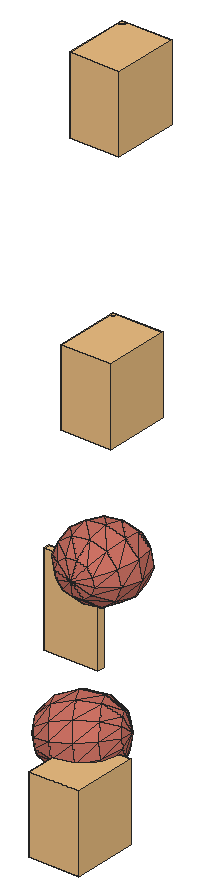
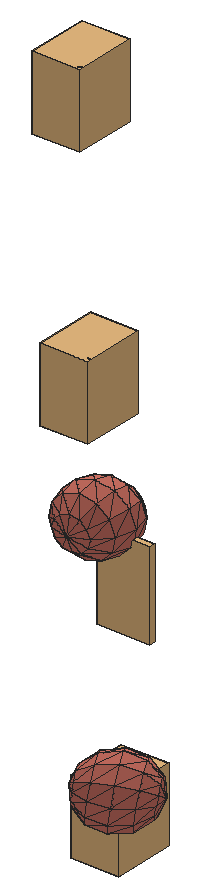
# SketchUp Ruby script. Lengths in inches.
U = 1.inch
M = Sketchup.active_model
def pt(a) = Geom::Point3d.new(a.map { |v| v * U })
def face(e, loops, mat)
  f = e.add_face(loops[0].map { |a| pt(a) })
  loops[1..].each { |l| e.add_face(l.map { |a| pt(a) }).erase! }
  f.material = f.back_material = mat if mat
  f
end
# faces: each face lists its corners as indices into pts; further lists are holes
def faces(e, pts, list, mat = nil) = list.each { |f| face(e, (f[0].is_a?(Array) ? f : [f]).map { |l| l.map { |i| pts[i] } }, mat) }
# xy, xz, yz: faces in a plane at the given z, y or x. An outline is a flat list of corners, or four numbers for a rectangle; further outlines are holes
def ring(l) = l.size == 4 ? [[l[0], l[1]], [l[2], l[1]], [l[2], l[3]], [l[0], l[3]]] : l.each_slice(2).to_a
def flat(e, list, mat, &to3) = list.each { |f| face(e, (f[0].is_a?(Array) ? f : [f]).map { |l| ring(l).map { |u, v| to3.(u, v) } }, mat) }
def xy(e, z, list, mat = nil) = flat(e, list, mat) { |x, y| [x, y, z] }
def xz(e, y, list, mat = nil) = flat(e, list, mat) { |x, z| [x, y, z] }
def yz(e, x, list, mat = nil) = flat(e, list, mat) { |y, z| [x, y, z] }
def lines(e, pts, list) = list.each { |a, b| e.add_line(pt(pts[a]), pt(pts[b])) }
# prism: a flat outline (further loops are holes) pulled along v
def prism(e, loops, v, mat = nil)
  f = face(e, loops, mat); d = Geom::Vector3d.new(v.map { |x| x * U })
  f.pushpull(f.normal.samedirection?(d) ? d.length : -d.length)
end
def box(e, o, s, mat = nil) = prism(e, [[o, [o[0] + s[0], o[1], o[2]], [o[0] + s[0], o[1] + s[1], o[2]], [o[0], o[1] + s[1], o[2]]]], [0, 0, s[2]], mat)
def at(x, y, z, deg = 0) = Geom::Transformation.translation(pt([x, y, z])) * Geom::Transformation.rotation(ORIGIN, Z_AXIS, deg.degrees)
def axes(o, x, y, z) = Geom::Transformation.new([*x, 0, *y, 0, *z, 0, *pt(o).to_a, 1])
def part(name) = M.definitions.add(name)
# library, detail: a bought-in or finely detailed component or shape, given as its bounding box
def library(name, o, s) = part(name).tap { |d| box(d.entities, o, s) }
def detail(e, o, s) = box(e.add_group.entities, o, s)
def put(e, d, t, mat = nil) = e.add_instance(d, t).tap { |i| i.material = mat if mat }
def group(e, t, mat = nil) = e.add_group.tap { |g| g.transformation = t; g.material = mat if mat }.entities
root = M.entities
M.materials.add("green").color = [174, 139, 102]
M.materials.add("vio").color = [206, 114, 100]
c1 = library("3DGeom~127_Defintion",[-35.65,-500,-298.26],[71.3,1000,596.52])
c2 = part("3DGeom~128_Defintion")
p = [[1.79,-469.7,-298.26],[1.7,-500,-240.6],[-27.6,-477.32,-283.92],[31.13,-477.23,-283.76],[1.7,-500,-240.6],[1.79,-469.7,-298.26],
  [1.79,-469.7,-298.26],[-27.6,-477.32,-283.92],[-15.17,-471.75,-294.44],[31.13,-477.23,-283.76],[1.79,-469.7,-298.26],[18.74,-471.7,-294.35],
  [-27.6,-477.32,-283.92],[1.7,-500,-240.6],[-27.65,-492.47,-255.09],[-27.6,-477.32,-283.92],[-27.65,-492.47,-255.09],[-32.17,-484.9,-269.52],
  [31.09,-492.38,-254.93],[1.7,-500,-240.6],[31.13,-477.23,-283.76],[31.09,-492.38,-254.93],[31.13,-477.23,-283.76],[35.65,-484.8,-269.34],
  [1.7,-500,-240.6],[-15.25,-498,-244.5],[-27.65,-492.47,-255.09],[1.7,-500,-240.6],[31.09,-492.38,-254.93],[18.66,-497.94,-244.41],
  [-1.83,497.78,298.26],[-1.65,500,230.49],[-18.62,499.82,234.98],[-1.83,497.78,298.26],[15.29,499.875,235.07],[-1.65,500,230.49],
  [-1.83,497.78,298.26],[-18.62,499.82,234.98],[-31.0625,499.4,247.35],[-1.83,497.78,298.26],[27.67,499.49,247.51],[15.29,499.875,235.07],
  [-1.83,497.78,298.26],[-31.0625,499.4,247.35],[-35.65,498.84,264.28],[-1.83,497.78,298.26],[32.17,498.94,264.47],[27.67,499.49,247.51],
  [-1.83,497.78,298.26],[-35.65,498.84,264.28],[-31.15,498.29,281.24],[-1.83,497.78,298.26],[27.58,498.375,281.4],[32.17,498.94,264.47],
  [-1.83,497.78,298.26],[-31.15,498.29,281.24],[-18.77,497.9,293.67],[-1.83,497.78,298.26],[15.14,497.95,293.77],[27.58,498.375,281.4]]
faces(c2.entities,p,[[0,1,2],[3,4,5],[6,7,8],[9,10,11],[12,13,14],[15,16,17],[18,19,20],[21,22,23],
  [24,25,26],[27,28,29],[30,31,32],[33,34,35],[36,37,38],[39,40,41],[42,43,44],[45,46,47],
  [48,49,50],[51,52,53],[54,55,56],[57,58,59]],"green")
c3 = part("3DGeom~230_Defintion")
p = [[-248.9,29.76,-432.23],[1.27,34.79,-498.32],[1.59,-181.375,-452.05],[251.38,-156.7,-390.8125],[251.1,30.51,-430.88],[-249.48,208.89,-356.66],
  [0.6,241.64,-411.0625],[-249.48,208.89,-356.66],[-248.62,-157.45,-392.16],[1.49,-348.94,-284.65],[251.29,-301.82,-245.84],[-248.62,-157.45,-392.16],
  [-432.38,16.75,-250.32],[-248.62,-157.45,-392.16],[-432.71,120.17,-206.7],[-248.9,29.76,-432.23],[-432.38,16.75,-250.32],[-249.48,208.89,-356.66],
  [-248.9,29.76,-432.23],[433.81,-90.04,-224.86],[433.65,18.05,-247.99],[433.81,-90.04,-224.86],[250.52,209.64,-355.32],[433.65,18.05,-247.99],
  [251.1,30.51,-430.88],[250.52,209.64,-355.32],[-250.19,331.95,-185.71],[-249.48,208.89,-356.66],[-0.22,383.74,-213.67],[250.52,209.64,-355.32],
  [0.6,241.64,-411.0625],[-250.19,331.95,-185.71],[-0.22,383.74,-213.67],[-248.62,-157.45,-392.16],[-248.71,-302.57,-247.1875],[-432.22,-91.34,-227.19],
  [-248.62,-157.45,-392.16],[-248.71,-302.57,-247.1875],[-432.38,16.75,-250.32],[-248.62,-157.45,-392.16],[-432.22,-91.34,-227.19],[251.38,-156.7,-390.8125],
  [433.76,-173.82,-141.16],[251.29,-301.82,-245.84],[251.38,-156.7,-390.8125],[433.81,-90.04,-224.86],[-433.125,191.22,-108],[-250.19,331.95,-185.71],
  [250.52,209.64,-355.32],[433.31,121.47,-204.37],[433.65,18.05,-247.99],[249.81,332.7,-184.37],[250.52,209.64,-355.32],[-0.22,383.74,-213.67],
  [249.81,332.7,-184.37],[250.52,209.64,-355.32],[-248.71,-302.57,-247.1875],[1.49,-348.94,-284.65],[0.99,-423.01,-40.98],[1.49,-348.94,-284.65],
  [250.86,-365.97,-34.82],[1.49,-348.94,-284.65],[251.29,-301.82,-245.84],[-500,-0.75,-1.35],[433.65,18.05,-247.99],[500,0.75,1.35],
  [433.65,18.05,-247.99],[-248.71,-302.57,-247.1875],[-249.14,-366.71,-36.17],[-432.27,-175.12,-143.49],[-249.14,-366.71,-36.17],[251.29,-301.82,-245.84],
  [433.51,-210.86,-19.33],[250.86,-365.97,-34.82],[251.29,-301.82,-245.84],[-250.86,365.97,34.82],[-0.22,383.74,-213.67],[-250.19,331.95,-185.71],
  [-0.99,423.01,40.98],[-0.22,383.74,-213.67],[-250.86,365.97,34.82],[-0.22,383.74,-213.67],[432.9,192.52,-105.67],[249.81,332.7,-184.37],
  [-433.51,210.86,19.33],[-250.86,365.97,34.82],[249.14,366.71,36.17],[249.81,332.7,-184.37],[249.14,366.71,36.17],[-432.52,-212.16,-21.66],
  [432.52,212.16,21.66],[249.14,366.71,36.17],[-249.14,-366.71,-36.17],[0.22,-383.74,213.67],[250.19,-331.95,185.71],[250.19,-331.95,185.71],
  [-249.14,-366.71,-36.17],[-249.81,-332.7,184.37],[-249.81,-332.7,184.37],[250.86,-365.97,-34.82],[433.125,-191.22,108],[250.19,-331.95,185.71],
  [250.86,-365.97,-34.82],[-432.9,-192.52,105.67],[-433.3125,-121.47,204.37],[-433.65,-18.05,247.99],[-433.81,90.04,224.86],[-433.76,173.82,141.16],
  [432.71,-120.17,206.7],[432.38,-16.75,250.32],[432.22,91.34,227.19],[432.38,-16.75,250.32],[432.27,175.12,143.49],[248.71,302.57,247.1875],
  [248.71,302.57,247.1875],[249.14,366.71,36.17],[-251.29,301.82,245.84],[-251.29,301.82,245.84],[-250.86,365.97,34.82],[-1.49,348.94,284.65],
  [248.71,302.57,247.1875],[-251.29,301.82,245.84],[-250.52,-209.64,355.32],[250.19,-331.95,185.71],[248.62,157.45,392.16],[248.62,157.45,392.16],
  [248.71,302.57,247.1875],[-249.81,-332.7,184.37],[-0.6,-241.64,411.0625],[-249.81,-332.7,184.37],[-0.6,-241.64,411.0625],[-250.52,-209.64,355.32],
  [0.22,-383.74,213.67],[250.19,-331.95,185.71],[249.48,-208.89,356.66],[250.19,-331.95,185.71],[249.48,-208.89,356.66],[-251.1,-30.51,430.88],
  [-251.1,-30.51,430.88],[249.48,-208.89,356.66],[432.38,-16.75,250.32],[0.22,-383.74,213.67],[-0.6,-241.64,411.0625],[-433.65,-18.05,247.99],
  [-251.38,156.7,390.8125],[-433.81,90.04,224.86],[-251.38,156.7,390.8125],[248.9,-29.76,432.23],[432.22,91.34,227.19],[248.62,157.45,392.16],
  [432.38,-16.75,250.32],[432.22,91.34,227.19],[-251.38,156.7,390.8125],[-1.49,348.94,284.65],[-251.29,301.82,245.84],[-1.59,181.375,452.05],
  [248.71,302.57,247.1875],[248.71,302.57,247.1875],[-1.49,348.94,284.65],[-433.65,-18.05,247.99],[-251.1,-30.51,430.88],[-251.38,156.7,390.8125],
  [249.48,-208.89,356.66],[432.38,-16.75,250.32],[248.9,-29.76,432.23],[-251.38,156.7,390.8125],[-1.49,348.94,284.65],[-250.52,-209.64,355.32],
  [-1.27,-34.79,498.32],[-250.52,-209.64,355.32],[-251.38,156.7,390.8125]]
faces(c3.entities,p,[[0,1,2],[1,3,2],[1,4,3],[5,1,0],[6,4,1],[7,6,1],[8,2,9],[2,10,9],
  [2,3,10],[0,2,11],[12,0,13],[14,15,16],[14,17,18],[4,19,3],[4,20,21],[22,23,24],
  [6,25,4],[26,6,27],[28,29,30],[31,32,6],[33,9,34],[35,36,37],[38,39,40],[41,42,43],
  [44,45,42],[46,17,14],[46,47,17],[48,49,50],[51,49,52],[53,54,55],[56,57,58],[59,60,58],
  [61,62,60],[16,35,63],[14,16,63],[45,64,65],[66,49,65],[67,58,68],[69,37,70],[35,37,69],
  [71,72,73],[74,42,72],[35,69,63],[42,45,65],[75,76,77],[78,54,79],[80,78,81],[46,14,63],
  [49,82,65],[83,82,49],[84,47,46],[84,85,47],[86,82,87],[78,88,54],[69,70,89],[69,89,63],
  [72,42,65],[84,46,63],[82,90,65],[91,90,82],[92,58,93],[58,94,93],[58,60,95],[96,93,97],
  [89,70,98],[99,100,101],[102,72,100],[89,98,103],[89,103,63],[100,72,65],[103,104,63],[104,105,63],
  [105,106,63],[107,84,63],[106,107,63],[108,100,65],[109,108,65],[110,111,65],[112,110,65],[90,112,65],
  [107,85,84],[113,112,90],[114,90,115],[107,116,85],[117,78,118],[119,120,88],[119,88,78],[121,119,78],
  [103,98,122],[103,122,104],[123,100,108],[106,116,107],[124,110,112],[125,112,126],[127,93,128],[129,130,131],
  [132,133,134],[135,108,136],[104,122,137],[104,138,105],[139,108,140],[141,134,142],[143,144,145],[106,146,116],
  [147,148,149],[147,150,151],[152,153,154],[155,149,156],[155,157,158],[159,160,161],[162,163,164],[165,155,166],
  [167,142,168],[169,168,160],[142,134,147],[160,155,170],[168,149,155],[168,147,149],[142,147,168],[160,168,155]],"vio")
c4 = library("3DGeom~148_Defintion",[-424.75,-500,-323.76],[849.5,1000,647.52])
c5 = part("3DGeom~149_Defintion")
p = [[-419.66,479.4,-302.56],[-386.2,481.32,-323.76],[-405.55,478.95,-317.48],[-419.66,479.4,-302.56],[-366.78,485.875,-319.73],[-386.2,481.32,-323.76],
  [-419.66,479.4,-302.56],[-352.51,491.39,-306.47],[-366.78,485.875,-319.73],[-419.66,479.4,-302.56],[-347.21,496.4,-287.52],[-352.51,491.39,-306.47],
  [-419.66,479.4,-302.56],[-424.75,482.55,-283.01],[-419.44,487.56,-264.0625],[-419.66,479.4,-302.56],[-366.41,500,-253.05],[-352.3,499.55,-267.97],
  [-419.66,479.4,-302.56],[-352.3,499.55,-267.97],[-347.21,496.4,-287.52],[-419.66,479.4,-302.56],[-405.17,493.08,-250.79],[-385.76,497.63,-246.76],
  [-419.66,479.4,-302.56],[-385.76,497.63,-246.76],[-366.41,500,-253.05],[-419.66,479.4,-302.56],[-419.44,487.56,-264.0625],[-405.17,493.08,-250.79],
  [368.25,-500,278.25],[381.22,-498.52,262.42],[397.44,-490.86,253.62],[422.57,-466.35,264.06],[368.25,-500,278.25],[397.44,-490.86,253.62],
  [422.57,-466.35,264.06],[397.44,-490.86,253.62],[412.58,-479.09,254.22],[418.52,-450.97,299.13],[368.25,-500,278.25],[422.57,-466.35,264.06],
  [422.57,-466.35,264.06],[424.75,-456.06,280.5],[368.25,-500,278.25],[364.2,-484.62,313.32],[362.02,-494.91,296.88],[364.2,-484.62,313.32],
  [368.25,-500,278.25],[389.33,-460.11,323.76],[389.33,-460.11,323.76],[368.25,-500,278.25],[389.33,-460.11,323.76],[405.55,-452.45,314.97],
  [364.2,-484.62,313.32],[389.33,-460.11,323.76],[374.19,-471.88,323.16]]
faces(c5.entities,p,[[0,1,2],[3,4,5],[6,7,8],[9,10,11],[12,13,14],[15,16,17],[18,19,20],[21,22,23],
  [24,25,26],[27,28,29],[30,31,32],[33,34,35],[36,37,38],[39,40,41],[39,42,43],[44,45,46],
  [47,48,49],[50,51,39],[52,39,53],[54,55,56]],"green")
c6 = library("3DGeom~140_Defintion",[-424.75,-500,-323.76],[849.5,1000,647.52])
c7 = part("3DGeom~141_Defintion")
p = [[-419.66,479.4,-302.56],[-386.2,481.32,-323.76],[-405.55,478.95,-317.48],[-419.66,479.4,-302.56],[-366.78,485.875,-319.73],[-386.2,481.32,-323.76],
  [-419.66,479.4,-302.56],[-352.51,491.39,-306.47],[-366.78,485.875,-319.73],[-419.66,479.4,-302.56],[-347.21,496.4,-287.52],[-352.51,491.39,-306.47],
  [-419.66,479.4,-302.56],[-424.75,482.55,-283.01],[-419.44,487.56,-264.0625],[-419.66,479.4,-302.56],[-366.41,500,-253.05],[-352.3,499.55,-267.97],
  [-419.66,479.4,-302.56],[-352.3,499.55,-267.97],[-347.21,496.4,-287.52],[-419.66,479.4,-302.56],[-405.17,493.08,-250.79],[-385.76,497.63,-246.76],
  [-419.66,479.4,-302.56],[-385.76,497.63,-246.76],[-366.41,500,-253.05],[-419.66,479.4,-302.56],[-419.44,487.56,-264.0625],[-405.17,493.08,-250.79],
  [368.25,-500,278.25],[381.22,-498.52,262.42],[397.44,-490.86,253.62],[422.57,-466.35,264.06],[368.25,-500,278.25],[397.44,-490.86,253.62],
  [422.57,-466.35,264.06],[397.44,-490.86,253.62],[412.58,-479.09,254.22],[418.52,-450.97,299.13],[368.25,-500,278.25],[422.57,-466.35,264.06],
  [422.57,-466.35,264.06],[424.75,-456.06,280.5],[368.25,-500,278.25],[364.2,-484.62,313.32],[362.02,-494.91,296.88],[364.2,-484.62,313.32],
  [368.25,-500,278.25],[389.33,-460.11,323.76],[389.33,-460.11,323.76],[368.25,-500,278.25],[389.33,-460.11,323.76],[405.55,-452.45,314.97],
  [364.2,-484.62,313.32],[389.33,-460.11,323.76],[374.19,-471.88,323.16]]
faces(c7.entities,p,[[0,1,2],[3,4,5],[6,7,8],[9,10,11],[12,13,14],[15,16,17],[18,19,20],[21,22,23],
  [24,25,26],[27,28,29],[30,31,32],[33,34,35],[36,37,38],[39,40,41],[39,42,43],[44,45,46],
  [47,48,49],[50,51,39],[52,39,53],[54,55,56]],"green")
c8 = library("3DGeom~144_Defintion",[-424.75,-500,-323.76],[849.5,1000,647.52])
c9 = part("3DGeom~145_Defintion")
p = [[-419.66,479.4,-302.56],[-386.2,481.32,-323.76],[-405.55,478.95,-317.48],[-419.66,479.4,-302.56],[-366.78,485.875,-319.73],[-386.2,481.32,-323.76],
  [-419.66,479.4,-302.56],[-352.51,491.39,-306.47],[-366.78,485.875,-319.73],[-419.66,479.4,-302.56],[-347.21,496.4,-287.52],[-352.51,491.39,-306.47],
  [-419.66,479.4,-302.56],[-424.75,482.55,-283.01],[-419.44,487.56,-264.0625],[-419.66,479.4,-302.56],[-366.41,500,-253.05],[-352.3,499.55,-267.97],
  [-419.66,479.4,-302.56],[-352.3,499.55,-267.97],[-347.21,496.4,-287.52],[-419.66,479.4,-302.56],[-405.17,493.08,-250.79],[-385.76,497.63,-246.76],
  [-419.66,479.4,-302.56],[-385.76,497.63,-246.76],[-366.41,500,-253.05],[-419.66,479.4,-302.56],[-419.44,487.56,-264.0625],[-405.17,493.08,-250.79],
  [368.25,-500,278.25],[381.22,-498.52,262.42],[397.44,-490.86,253.62],[422.57,-466.35,264.06],[368.25,-500,278.25],[397.44,-490.86,253.62],
  [422.57,-466.35,264.06],[397.44,-490.86,253.62],[412.58,-479.09,254.22],[418.52,-450.97,299.13],[368.25,-500,278.25],[422.57,-466.35,264.06],
  [422.57,-466.35,264.06],[424.75,-456.06,280.5],[368.25,-500,278.25],[364.2,-484.62,313.32],[362.02,-494.91,296.88],[364.2,-484.62,313.32],
  [368.25,-500,278.25],[389.33,-460.11,323.76],[389.33,-460.11,323.76],[368.25,-500,278.25],[389.33,-460.11,323.76],[405.55,-452.45,314.97],
  [364.2,-484.62,313.32],[389.33,-460.11,323.76],[374.19,-471.88,323.16]]
faces(c9.entities,p,[[0,1,2],[3,4,5],[6,7,8],[9,10,11],[12,13,14],[15,16,17],[18,19,20],[21,22,23],
  [24,25,26],[27,28,29],[30,31,32],[33,34,35],[36,37,38],[39,40,41],[39,42,43],[44,45,46],
  [47,48,49],[50,51,39],[52,39,53],[54,55,56]],"green")
c10 = part("3DGeom~236_Defintion")
p = [[-0.24,-111.46,-482.47],[-247.71,40.8125,-431.68],[-3.37,-2.64,-500],[241.88,-45.39,-434.35],[50.53,96.35,-484.34],[-154.36,212.27,-404.56],
  [147.01,158.99,-439.69],[12.76,320.76,-327.23],[59.09,-200.9375,-436.46],[-242.29,-147.66,-401.32],[260.24,168.49,-378.02],[208.87,337.23,-220.41],
  [208.87,337.23,-220.41],[-139.53,-302.65,-321.625],[158.71,-247.11,-374.29],[271.93,-237.61,-312.62],[368.42,-174.96,-267.97],[422.32,-75.98,-252.31],
  [419.18,32.84,-269.83],[359.86,122.32,-315.85],[-242.29,-147.66,-401.32],[-425.68,73.33,-247.69],[-247.71,40.8125,-431.68],[-425.68,73.33,-247.69],
  [-317.89,271.31,-216.37],[-317.89,271.31,-216.37],[-154.36,212.27,-404.56],[-317.89,271.31,-216.37],[-124.92,396.59,-127.08],[-154.36,212.27,-404.56],
  [12.76,320.76,-327.23],[-139.53,-302.65,-321.625],[-419.42,-144.29,-212.64],[-242.29,-147.66,-401.32],[-242.29,-147.66,-401.32],[-425.68,73.33,-247.69],
  [260.24,168.49,-378.02],[381.41,257.26,-112.72],[359.86,122.32,-315.85],[260.24,168.49,-378.02],[208.87,337.23,-220.41],[33.01,-382.62,-213.94],
  [271.93,-237.61,-312.62],[33.01,-382.62,-213.94],[158.71,-247.11,-374.29],[12.76,320.76,-327.23],[101.53,415.61,-3.73],[12.76,320.76,-327.23],
  [208.87,337.23,-220.41],[33.01,-382.62,-213.94],[-300.77,-323.26,-120.61],[-139.53,-302.65,-321.625],[-139.53,-302.65,-321.625],[-300.77,-323.26,-120.61],
  [359.86,122.32,-315.85],[484.17,102.27,-33.02],[419.18,32.84,-269.83],[359.86,122.32,-315.85],[271.93,-237.61,-312.62],[229.12,-366.15,-107.12],
  [33.01,-382.62,-213.94],[368.42,-174.96,-267.97],[229.12,-366.15,-107.12],[271.93,-237.61,-312.62],[419.18,32.84,-269.83],[489.59,-86.2,-2.67],
  [419.18,32.84,-269.83],[422.32,-75.98,-252.31],[368.42,-174.96,-267.97],[396.24,-257.66,-29.79],[229.12,-366.15,-107.12],[422.32,-75.98,-252.31],
  [368.42,-174.96,-267.97],[422.32,-75.98,-252.31],[-489.59,86.2,2.67],[-425.68,73.33,-247.69],[-425.68,73.33,-247.69],[-396.24,257.66,29.79],
  [-425.68,73.33,-247.69],[-396.24,257.66,29.79],[-317.89,271.31,-216.37],[208.87,337.23,-220.41],[300.77,323.26,120.61],[381.41,257.26,-112.72],
  [208.87,337.23,-220.41],[300.77,323.26,120.61],[-396.24,257.66,29.79],[-229.12,366.15,107.12],[33.01,-382.62,-213.94],[-101.53,-415.61,3.73],
  [-300.77,-323.26,-120.61],[33.01,-382.62,-213.94],[-484.17,-102.27,33.02],[-33.01,382.62,213.94],[-381.41,-257.26,112.72],[-300.77,-323.26,-120.61],
  [-381.41,-257.26,112.72],[419.42,144.29,212.64],[300.77,323.26,120.61],[124.92,-396.59,127.08],[396.24,-257.66,-29.79],[425.68,-73.33,247.69],
  [396.24,-257.66,-29.79],[317.89,-271.31,216.37],[317.89,-271.31,216.37],[139.53,302.65,321.625],[139.53,302.65,321.625],[300.77,323.26,120.61],
  [-422.32,75.98,252.31],[-368.42,174.96,267.97],[-396.24,257.66,29.79],[-208.87,-337.23,220.41],[-381.41,-257.26,112.72],[-396.24,257.66,29.79],
  [-271.93,237.61,312.62],[-396.24,257.66,29.79],[-271.93,237.61,312.62],[-229.12,366.15,107.12],[-419.18,-32.84,269.83],[-271.93,237.61,312.62],
  [-158.71,247.11,374.29],[-158.71,247.11,374.29],[-208.87,-337.23,220.41],[-359.86,-122.32,315.85],[242.29,147.66,401.32],[139.53,302.65,321.625],
  [-12.76,-320.76,327.23],[317.89,-271.31,216.37],[247.71,-40.8125,431.68],[247.71,-40.8125,431.68],[-33.01,382.62,213.94],[-158.71,247.11,374.29],
  [-59.09,200.94,436.46],[-33.01,382.62,213.94],[139.53,302.65,321.625],[317.89,-271.31,216.37],[154.36,-212.27,404.56],[425.68,-73.33,247.69],
  [154.36,-212.27,404.56],[317.89,-271.31,216.37],[-208.87,-337.23,220.41],[-260.24,-168.49,378.02],[-12.76,-320.76,327.23],[-260.24,-168.49,378.02],
  [-208.87,-337.23,220.41],[425.68,-73.33,247.69],[247.71,-40.8125,431.68],[-422.32,75.98,252.31],[-419.18,-32.84,269.83],[-241.88,45.39,434.35],
  [-368.42,174.96,267.97],[-422.32,75.98,252.31],[-271.93,237.61,312.62],[-368.42,174.96,267.97],[-419.18,-32.84,269.83],[-359.86,-122.32,315.85],
  [-271.93,237.61,312.62],[-359.86,-122.32,315.85],[-260.24,-168.49,378.02],[139.53,302.65,321.625],[0.24,111.46,482.47],[139.53,302.65,321.625],
  [242.29,147.66,401.32],[-12.76,-320.76,327.23],[-147.01,-158.99,439.69],[-260.24,-168.49,378.02],[-12.76,-320.76,327.23],[-260.24,-168.49,378.02],
  [242.29,147.66,401.32],[3.37,2.64,500],[242.29,147.66,401.32],[-50.53,-96.35,484.34]]
faces(c10.entities,p,[[0,1,2],[0,2,3],[2,4,3],[2,1,5],[2,5,4],[4,6,3],[4,5,7],[4,7,6],
  [8,9,0],[8,0,3],[0,9,1],[6,10,3],[6,7,11],[6,12,10],[8,13,9],[14,13,8],
  [14,8,3],[15,14,3],[16,15,3],[17,16,3],[18,17,3],[19,18,3],[10,19,3],[20,21,22],
  [1,23,24],[1,25,5],[26,27,28],[29,28,30],[31,32,33],[34,32,35],[36,37,38],[39,40,37],
  [14,41,13],[42,43,44],[45,28,46],[47,46,48],[49,50,51],[52,53,32],[54,55,56],[57,37,55],
  [58,59,60],[61,62,63],[64,55,65],[66,65,67],[68,69,70],[71,69,72],[73,65,69],[32,74,75],
  [76,74,77],[78,79,80],[81,82,83],[84,46,85],[27,86,87],[27,87,28],[88,89,90],[59,89,91],
  [53,92,32],[32,92,74],[28,87,93],[28,93,46],[89,94,95],[53,96,92],[37,97,55],[37,98,97],
  [59,99,89],[100,99,59],[55,101,65],[55,97,101],[102,103,99],[65,104,69],[46,93,105],[46,106,107],
  [65,101,104],[92,108,74],[74,108,109],[74,109,110],[89,111,112],[99,111,89],[113,109,114],[115,116,117],
  [96,118,92],[92,118,108],[87,119,120],[87,121,93],[122,123,96],[96,123,118],[98,124,97],[98,125,124],
  [99,126,111],[127,126,99],[97,128,101],[97,124,129],[130,131,132],[133,132,134],[135,136,126],[137,138,139],
  [140,141,123],[142,143,144],[145,146,138],[147,148,149],[150,151,149],[152,153,149],[154,155,149],[131,156,149],
  [157,158,149],[159,132,160],[161,160,162],[163,164,165],[138,164,166],[132,131,149],[167,164,149],[168,169,146],
  [170,160,169],[138,171,164],[146,171,138],[146,169,171],[164,171,149],[171,169,149],[169,160,149],[160,132,149]],"vio")
g1 = group(root,at(15.3125,134.49,26.21))
put(g1,c1,axes([-2.06,0.6,10.86],[0,0.00044,0],[0,0,-0.00044],[-0.00044,0,0]),"green")
put(g1,c2,axes([-2.06,0.6,10.86],[0,0.00044,0],[0,0,-0.00044],[-0.00044,0,0]),"green")
g2 = group(root,at(15.3125,134.49,26.21))
put(g2,c3,axes([-1.92,0.6,11.11],[0,0.00039,0],[0,0,-0.00039],[-0.00039,0,0]),"vio")
g3 = group(root,at(15.3125,134.49,26.21))
put(g3,c4,axes([-2.125,0.72,9.92],[0,0.00037,0],[0,0,-0.00037],[-0.00037,0,0]),"green")
put(g3,c5,axes([-2.125,0.72,9.92],[0,0.00037,0],[0,0,-0.00037],[-0.00037,0,0]),"green")
g4 = group(root,at(15.3125,134.49,26.21))
put(g4,c6,axes([-1.93,0.72,13.1],[0,0.00037,0],[0,0,-0.00037],[-0.00037,0,0]),"green")
put(g4,c7,axes([-1.93,0.72,13.1],[0,0.00037,0],[0,0,-0.00037],[-0.00037,0,0]),"green")
g5 = group(root,at(15.3125,134.49,26.21))
put(g5,c8,axes([-1.98,0.73,11.8125],[0,0.00037,0],[0,0,-0.00037],[-0.00037,0,0]),"green")
put(g5,c9,axes([-1.98,0.73,11.8125],[0,0.00037,0],[0,0,-0.00037],[-0.00037,0,0]),"green")
g6 = group(root,at(15.3125,134.49,26.21))
put(g6,c10,axes([-2.25,0.89,10.125],[0,0.00039,0],[0,0,-0.00039],[-0.00039,0,0]),"vio")
